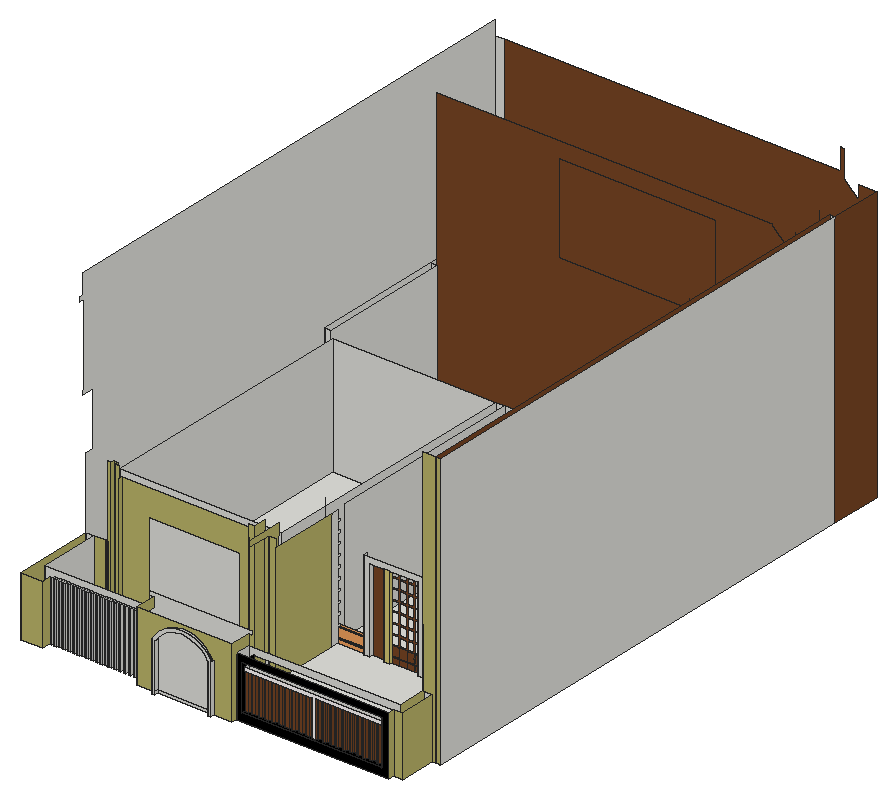
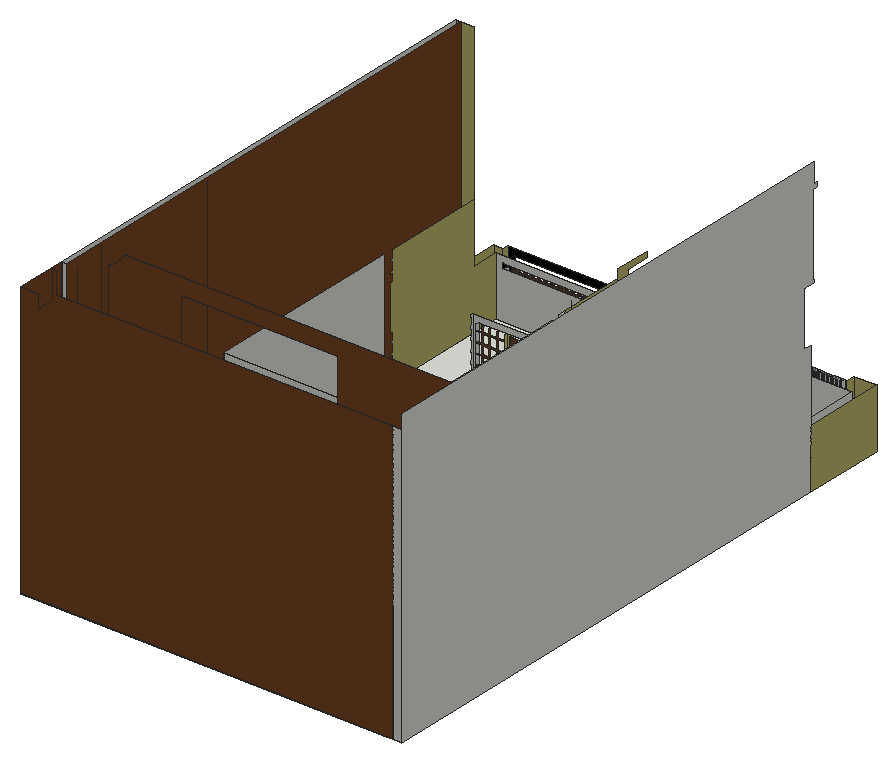
# SketchUp Ruby script. Lengths in inches.
U = 1.inch
M = Sketchup.active_model
def pt(a) = Geom::Point3d.new(a.map { |v| v * U })
def face(e, loops, mat)
  f = e.add_face(loops[0].map { |a| pt(a) })
  loops[1..].each { |l| e.add_face(l.map { |a| pt(a) }).erase! }
  f.material = f.back_material = mat if mat
  f
end
# faces: each face lists its corners as indices into pts; further lists are holes
def faces(e, pts, list, mat = nil) = list.each { |f| face(e, (f[0].is_a?(Array) ? f : [f]).map { |l| l.map { |i| pts[i] } }, mat) }
# xy, xz, yz: faces in a plane at the given z, y or x. An outline is a flat list of corners, or four numbers for a rectangle; further outlines are holes
def ring(l) = l.size == 4 ? [[l[0], l[1]], [l[2], l[1]], [l[2], l[3]], [l[0], l[3]]] : l.each_slice(2).to_a
def flat(e, list, mat, &to3) = list.each { |f| face(e, (f[0].is_a?(Array) ? f : [f]).map { |l| ring(l).map { |u, v| to3.(u, v) } }, mat) }
def xy(e, z, list, mat = nil) = flat(e, list, mat) { |x, y| [x, y, z] }
def xz(e, y, list, mat = nil) = flat(e, list, mat) { |x, z| [x, y, z] }
def yz(e, x, list, mat = nil) = flat(e, list, mat) { |y, z| [x, y, z] }
def lines(e, pts, list) = list.each { |a, b| e.add_line(pt(pts[a]), pt(pts[b])) }
# prism: a flat outline (further loops are holes) pulled along v
def prism(e, loops, v, mat = nil)
  f = face(e, loops, mat); d = Geom::Vector3d.new(v.map { |x| x * U })
  f.pushpull(f.normal.samedirection?(d) ? d.length : -d.length)
end
def box(e, o, s, mat = nil) = prism(e, [[o, [o[0] + s[0], o[1], o[2]], [o[0] + s[0], o[1] + s[1], o[2]], [o[0], o[1] + s[1], o[2]]]], [0, 0, s[2]], mat)
def at(x, y, z, deg = 0) = Geom::Transformation.translation(pt([x, y, z])) * Geom::Transformation.rotation(ORIGIN, Z_AXIS, deg.degrees)
def axes(o, x, y, z) = Geom::Transformation.new([*x, 0, *y, 0, *z, 0, *pt(o).to_a, 1])
def part(name) = M.definitions.add(name)
# library, detail: a bought-in or finely detailed component or shape, given as its bounding box
def library(name, o, s) = part(name).tap { |d| box(d.entities, o, s) }
def detail(e, o, s) = box(e.add_group.entities, o, s)
def put(e, d, t, mat = nil) = e.add_instance(d, t).tap { |i| i.material = mat if mat }
def group(e, t, mat = nil) = e.add_group.tap { |g| g.transformation = t; g.material = mat if mat }.entities
root = M.entities
M.materials.add("[0010_Snow]").color = [255, 250, 250]
M.materials.add("[0037_SandyBrown]").color = [244, 164, 96]
M.materials.add("[0057_DarkKhaki]").color = [189, 183, 107]
M.materials.add("[0131_Silver]").color = [192, 192, 192]
M.materials.add("[0137_Black]").color = [0, 0, 0]
M.materials.add("[Wood Board Cork]").color = [215, 201, 115]
M.materials.add("[Wood Veneer 01]").color = [120, 70, 37]
xy(root,0,[[163.64,1.8125,166.64,1.8125,166.64,4.8125,219.7,4.8125,219.7,1.8125,222.7,1.8125,222.7,4.8125,241.27,4.8125,241.27,25.8125,43.3125,25.8125,43.3125,4.8125,50.69,4.8125,50.69,13.8125,53.49,13.8125,53.49,16.8125,55.32,16.8125,55.32,13.8125,58.12,13.8125,58.12,16.8125,145.98,16.8125,145.98,4.8125,163.64,4.8125],[28.5625,4.8125,28.5625,87.625,36.25,87.625,36.25,25.8125,43.3125,25.8125,43.3125,4.8125],[241.27,10.8125,241.27,25.8125,394.3125,25.8125,394.3125,54.1875,403.3125,54.1875,403.3125,16.8125,394.3125,16.8125,394.3125,10.8125],[59.94,13.8125,62.74,16.8125],[64.57,13.8125,67.37,16.8125],
  [69.19,13.8125,71.99,16.8125],[73.82,13.8125,76.62,16.8125],[78.44,13.8125,81.24,16.8125],[83.07,13.8125,85.87,16.8125],[87.69,13.8125,90.49,16.8125],
  [92.32,13.8125,95.12,16.8125],[96.94,13.8125,99.74,16.8125],[101.57,13.8125,104.37,16.8125],[106.19,13.8125,108.99,16.8125],[110.82,13.8125,113.62,16.8125],
  [115.44,13.8125,118.24,16.8125],[120.07,13.8125,122.87,16.8125],[125.13,13.8125,127.93,16.8125],[130.19,13.8125,132.99,16.8125],[135.25,13.8125,138.06,16.8125],
  [140.32,13.8125,143.12,16.8125],[145.38,13.8125,145.98,16.8125],[36.25,25.8125,43.3125,87.625],[43.3125,25.8125,394.3125,25.8125,394.3125,155.75,314.53,155.75,314.53,154.75,308.53,154.75,308.53,157.75,279.73,157.75,279.73,154.75,274.66,154.75,274.66,157.75,260.53,157.75,260.53,154.75,254.53,154.75,254.53,155.75,227.125,155.75,227.125,77.875,220.06,77.875,220.06,90.625,205.65,90.625,205.65,77.875,199.44,77.875,199.44,90.625,61.7,90.625,61.7,87.625,57.59,87.625,57.59,90.625,53.48,90.625,53.48,87.625,43.3125,87.625],[394.3125,54.1875,395.5625,54.1875,395.5625,376.8125,43.3125,376.8125,43.3125,87.625,47.8125,87.625,47.8125,90.625,50.0625,90.625,50.0625,87.625,53.48,87.625,53.48,90.625,57.59,90.625,57.59,87.625,61.7,87.625,61.7,90.625,199.44,90.625,199.44,77.875,203.15,77.875,203.15,90.625,220.06,90.625,220.06,148.375,225.0625,148.375,225.0625,367.8125,216.0625,367.8125,216.0625,99.625,52.3125,99.625,52.3125,367.8125,394.3125,367.8125],
  [395.5625,54.1875,403.3125,376.8125],[403.3125,54.1875,406.875,376.8125],[406.875,54.1875,410.5,376.8125],[410.5,54.1875,410.5,376.8125,406.875,376.8125,406.875,550.125,410.875,550.125,410.875,54.1875],[410.875,54.1875,411.75,550.125],
  [203.15,77.875,205.65,90.625],[220.06,77.875,225.0625,90.625],[225.0625,77.875,227.125,90.625],[28.5625,87.625,28.5625,601.9375,37.25,601.9375,37.25,376.8125,43.3125,376.8125,43.3125,87.625],[220.06,90.625,225.0625,148.375],
  [225.0625,90.625,227.125,148.375],[52.3125,99.625,216.0625,367.8125],[225.0625,148.375,227.125,157.75],[254.53,154.75,260.53,157.75],[274.66,154.75,279.73,157.75],
  [308.53,154.75,314.53,157.75],[227.125,155.75,254.53,157.75],[314.53,155.75,394.3125,157.75],[225.0625,157.75,394.3125,158.8125],[225.0625,158.8125,394.3125,367.8125],
  [37.25,376.8125,43.3125,510.5],[43.3125,376.8125,395.5625,510.5],[395.5625,376.8125,403.3125,510.5],[403.3125,376.8125,406.875,550.125],[37.25,510.5,43.3125,601.9375],
  [43.3125,510.5,395.5625,550.125],[395.5625,510.5,403.3125,550.125],[43.3125,550.125,403.3125,601.9375],[403.3125,550.125,410.875,601.9375],[410.875,550.125,411.75,601.9375]])
xy(root,3.8125,[[227.125,155.75,254.53,157.75],[314.53,155.75,394.3125,157.75]],"[0037_SandyBrown]")
xy(root,5.97,[[227.125,155.75,254.53,157.75],[314.53,155.75,394.3125,157.75],[227.125,157.75,254.53,157.9375]])
xy(root,7.54,[[246.54,10.8125,387.24,10.8125,387.24,14.8125,385.6,14.8125,385.6,16.8125,381.54,16.8125,381.54,14.8125,378.85,14.8125,378.85,16.8125,374.79,16.8125,374.79,14.8125,372.1,14.8125,372.1,16.8125,368.04,16.8125,368.04,14.8125,365.35,14.8125,365.35,16.8125,361.29,16.8125,361.29,14.8125,358.6,14.8125,358.6,16.8125,354.54,16.8125,354.54,14.8125,351.85,14.8125,351.85,16.8125,347.79,16.8125,347.79,14.8125,345.1,14.8125,345.1,16.8125,341.04,16.8125,341.04,14.8125,338.35,14.8125,338.35,16.8125,334.29,16.8125,334.29,14.8125,331.6,14.8125,331.6,16.8125,327.54,16.8125,327.54,14.8125,324.85,14.8125,324.85,16.8125,320.79,16.8125,320.79,14.8125,318.91,14.8125,318.91,13.8125,314.71,13.8125,314.71,14.8125,314.04,14.8125,314.04,16.8125,311.35,16.8125,311.35,14.8125,307.29,14.8125,307.29,16.8125,304.6,16.8125,304.6,14.8125,300.54,14.8125,300.54,16.8125,297.85,16.8125,297.85,14.8125,293.79,14.8125,293.79,16.8125,291.1,16.8125,291.1,14.8125,287.04,14.8125,287.04,16.8125,284.35,16.8125,284.35,14.8125,280.29,14.8125,280.29,16.8125,277.6,16.8125,277.6,14.8125,273.54,14.8125,273.54,16.8125,270.85,16.8125,270.85,14.8125,266.79,14.8125,266.79,16.8125,264.1,16.8125,264.1,14.8125,260.04,14.8125,260.04,16.8125,257.35,16.8125,257.35,14.8125,253.29,14.8125,253.29,16.8125,250.6,16.8125,250.6,14.8125,246.54,14.8125]],"[0137_Black]")
xy(root,9.66,[[205.65,89.5625,220.06,90.625]])
xy(root,14.375,[[227.125,157.75,254.53,157.9375]])
xy(root,14.375,[[227.125,155.75,254.53,157.75],[314.53,155.75,394.3125,157.75]],"[0037_SandyBrown]")
xz(root,1.8125,[[163.64,0,166.64,0,166.64,48.36,169.3,52.43,173.07,56.4,177.5,59.64,182.43,62.03,187.71,63.5,193.17,63.99,198.63,63.5,203.91,62.03,208.85,59.64,213.27,56.4,217.05,52.43,219.7,48.36,219.7,0,222.7,0,222.7,49.25,219.41,54.29,215.26,58.67,210.4,62.22,204.98,64.85,199.17,66.46,193.17,67,187.17,66.46,181.37,64.85,175.94,62.22,171.08,58.67,166.93,54.29,163.64,49.25]])
xz(root,4.8125,[[166.64,0,219.7,3],[166.64,3,219.7,3,219.7,48.36,217.05,52.43,213.27,56.4,208.85,59.64,203.91,62.03,198.63,63.5,193.17,63.99,187.71,63.5,182.43,62.03,177.5,59.64,173.07,56.4,169.3,52.43,166.64,48.36]])
xz(root,4.8125,[[28.5625,0,50.69,60],[145.98,0,163.64,0,163.64,49.25,166.93,54.29,171.08,58.67,175.94,62.22,181.37,64.85,187.17,66.46,193.17,67,199.17,66.46,204.98,64.85,210.4,62.22,215.26,58.67,219.41,54.29,222.7,49.25,222.7,0,241.27,0,241.27,70.61,145.98,70.61]],"[0057_DarkKhaki]")
xz(root,10.8125,[[[241.27,0,394.3125,60],[246.54,7.54,387.24,53.24]]],"[0137_Black]")
xz(root,13.8125,[[314.71,7.54,318.91,7.54,318.91,44.24,387.24,44.24,387.24,48.11,246.54,48.11,246.54,44.24,314.71,44.24]],"[0010_Snow]")
xz(root,13.8125,[[50.69,0,53.49,60],[55.32,0,58.12,60],[59.94,0,62.74,60],[64.57,0,67.37,60],[69.19,0,71.99,60],
  [73.82,0,76.62,60],[78.44,0,81.24,60],[83.07,0,85.87,60],[87.69,0,90.49,60],[92.32,0,95.12,60],
  [96.94,0,99.74,60],[101.57,0,104.37,60],[106.19,0,108.99,60],[110.82,0,113.62,60],[115.44,0,118.24,60],
  [120.07,0,122.87,60],[125.13,0,127.93,60],[130.19,0,132.99,60],[135.25,0,138.06,60],[140.32,0,143.12,60],
  [145.38,0,145.98,60]],"[0131_Silver]")
xz(root,14.8125,[[246.54,7.54,250.6,44.24],[253.29,7.54,257.35,44.24],[260.04,7.54,264.1,44.24],[266.79,7.54,270.85,44.24],[273.54,7.54,277.6,44.24],
  [280.29,7.54,284.35,44.24],[287.04,7.54,291.1,44.24],[293.79,7.54,297.85,44.24],[300.54,7.54,304.6,44.24],[307.29,7.54,311.35,44.24],
  [314.04,7.54,314.71,44.24],[318.91,7.54,320.79,44.24],[324.85,7.54,327.54,44.24],[331.6,7.54,334.29,44.24],[338.35,7.54,341.04,44.24],
  [345.1,7.54,347.79,44.24],[351.85,7.54,354.54,44.24],[358.6,7.54,361.29,44.24],[365.35,7.54,368.04,44.24],[372.1,7.54,374.79,44.24],
  [378.85,7.54,381.54,44.24],[385.6,7.54,387.24,44.24]],"[Wood Veneer 01]")
xz(root,16.8125,[[59.94,0,62.74,60],[64.57,0,67.37,60],[69.19,0,71.99,60],[73.82,0,76.62,60],[78.44,0,81.24,60],
  [83.07,0,85.87,60],[87.69,0,90.49,60],[92.32,0,95.12,60],[96.94,0,99.74,60],[101.57,0,104.37,60],
  [106.19,0,108.99,60],[110.82,0,113.62,60],[115.44,0,118.24,60],[120.07,0,122.87,60],[125.13,0,127.93,60],
  [130.19,0,132.99,60],[135.25,0,138.06,60],[140.32,0,143.12,60],[145.38,0,145.98,60],[145.98,0,148.18,60],
  [314.71,7.54,318.1,44.24],[388.29,7.54,392.35,44.24]])
xz(root,16.8125,[[394.3125,0,403.3125,60]],"[0057_DarkKhaki]")
xz(root,16.8125,[[53.49,0,55.32,60],[58.12,0,59.94,60],[62.74,0,64.57,60],[67.37,0,69.19,60],[71.99,0,73.82,60],
  [76.62,0,78.44,60],[81.24,0,83.07,60],[85.87,0,87.69,60],[90.49,0,92.32,60],[95.12,0,96.94,60],
  [99.74,0,101.57,60],[104.37,0,106.19,60],[108.99,0,110.82,60],[113.62,0,115.44,60],[118.24,0,120.07,60],
  [122.87,0,125.13,60],[127.93,0,130.19,60],[132.99,0,135.25,60],[138.06,0,140.32,60],[143.12,0,145.38,60]],"[0131_Silver]")
xz(root,16.8125,[[250.6,7.54,253.29,44.24],[257.35,7.54,260.04,44.24],[264.1,7.54,266.79,44.24],[270.85,7.54,273.54,44.24],[277.6,7.54,280.29,44.24],
  [284.35,7.54,287.04,44.24],[291.1,7.54,293.79,44.24],[297.85,7.54,300.54,44.24],[304.6,7.54,307.29,44.24],[311.35,7.54,314.04,44.24],
  [320.79,7.54,324.85,44.24],[327.54,7.54,331.6,44.24],[334.29,7.54,338.35,44.24],[341.04,7.54,345.1,44.24],[347.79,7.54,351.85,44.24],
  [354.54,7.54,358.6,44.24],[361.29,7.54,365.35,44.24],[368.04,7.54,372.1,44.24],[374.79,7.54,378.85,44.24],[381.54,7.54,385.6,44.24]],"[Wood Veneer 01]")
xz(root,25.8125,[[36.25,0,36.25,60,145.98,60,145.98,70.61,142.42,70.61,142.42,74.1875,244.96,74.1875,244.96,70.75,241.27,70.75,241.27,0],[[241.27,0,394.3125,60],[246.54,48.11,387.24,53.24]]])
xz(root,54.1875,[[395.5625,0,403.3125,60]])
xz(root,54.1875,[[403.3125,0,406.875,0,406.875,276,394.3125,276,394.3125,60,403.3125,60],[406.875,0,411.75,276]],"[0057_DarkKhaki]")
xz(root,77.875,[[199.44,0,205.65,132],[220.06,0,227.125,128.6875]],"[0057_DarkKhaki]")
xz(root,87.625,[[28.5625,0,36.25,60]])
xz(root,87.625,[[36.25,0,47.8125,60],[47.8125,0,50.0625,60],[50.0625,0,53.48,132],[57.59,0,61.7,132]],"[0057_DarkKhaki]")
xz(root,89.5625,[[205.65,9.66,220.06,123.17]],"[0057_DarkKhaki]")
xz(root,90.625,[[47.8125,0,50.0625,60],[205.65,0,220.06,9.66]])
xz(root,90.625,[[53.48,0,57.59,132],[[61.7,0,199.44,120],[88.6875,15.35,180.5,93.6]]],"[0057_DarkKhaki]")
xz(root,99.625,[[52.3125,0,216.0625,120]])
xz(root,154.75,[[254.53,0,260.53,0,260.53,84,308.53,84,308.53,0,314.53,0,314.53,90,254.53,90]])
xz(root,154.75,[[274.66,0,279.73,84]],"[Wood Board Cork]")
xz(root,155.75,[[227.125,0,254.53,3.8125],[314.53,0,394.3125,3.8125],[227.125,5.97,254.53,14.375],[314.53,5.97,394.3125,14.375]],"[0037_SandyBrown]")
xz(root,157.75,[[225.0625,0,227.125,3.8125],[227.125,0,254.53,3.8125],[254.53,0,260.53,3.8125],[274.66,0,279.73,3.8125],[308.53,0,314.53,3.8125],
  [314.53,0,394.3125,3.8125],[225.0625,3.8125,227.125,5.97],[254.53,3.8125,260.53,5.97],[308.53,3.8125,314.53,5.97],[225.0625,5.97,227.125,14.375],
  [254.53,5.97,260.53,14.375],[274.66,5.97,279.73,14.375],[308.53,5.97,314.53,14.375],[314.53,5.97,394.3125,14.375],[225.0625,14.375,227.125,16.53],
  [254.53,14.375,260.53,16.53],[308.53,14.375,314.53,16.53]])
xz(root,157.75,[[227.125,3.8125,254.53,5.97],[314.53,3.8125,394.3125,5.97],[227.125,14.375,254.53,16.53],[314.53,14.375,394.3125,16.53]],"[0037_SandyBrown]")
xz(root,157.75,[[260.53,0,274.66,84],[279.73,0,286.72,5.28],[[286.72,0,287.41,0,287.41,5.28,295.09,5.28,295.09,0,295.95,0,295.95,5.28,302.05,5.28,302.05,0,302.96,0,302.96,5.28,308.53,5.28,308.53,6.47,302.96,6.47,302.96,15.84,308.53,15.84,308.53,17.03,302.96,17.03,302.96,25.59,308.53,25.59,308.53,26.78,302.96,26.78,302.96,35.97,308.53,35.97,308.53,37.15,302.96,37.15,302.96,46.34,308.53,46.34,308.53,47.53,302.96,47.53,302.96,56.72,308.53,56.72,308.53,57.9,302.96,57.9,302.96,67.09,308.53,67.09,308.53,68.28,302.96,68.28,302.96,77.47,308.53,77.47,308.53,78.65,302.96,78.65,302.96,84,302.05,84,302.05,78.65,295.95,78.65,295.95,84,295.09,84,295.09,78.65,287.41,78.65,287.41,84,286.72,84,286.72,78.65,279.73,78.65,279.73,77.47,286.72,77.47,286.72,68.28,279.73,68.28,279.73,67.09,286.72,67.09,286.72,57.9,279.73,57.9,279.73,56.72,286.72,56.72,286.72,47.53,279.73,47.53,279.73,46.34,286.72,46.34,286.72,37.15,279.73,37.15,279.73,35.97,286.72,35.97,286.72,26.78,279.73,26.78,279.73,25.59,286.72,25.59,286.72,17.03,279.73,17.03,279.73,15.84,286.72,15.84,286.72,6.47,279.73,6.47,279.73,5.28,286.72,5.28],[287.41,6.47,295.09,15.84],[287.41,68.28,295.09,77.47],[287.41,26.78,295.09,35.97],[287.41,47.53,295.09,56.72],[287.41,57.9,295.09,67.09],[287.41,37.15,295.09,46.34],[287.41,17.03,295.09,25.59],[295.95,6.47,302.05,15.84],[295.95,68.28,302.05,77.47],[295.95,26.78,302.05,35.97],[295.95,47.53,302.05,56.72],[295.95,57.9,302.05,67.09],[295.95,37.15,302.05,46.34],[295.95,17.03,302.05,25.59]],[287.41,0,295.09,5.28],[295.95,0,302.05,5.28],
  [302.96,0,308.53,5.28],[279.73,6.47,286.72,15.84],[287.41,6.47,295.09,15.84],[295.95,6.47,302.05,15.84],[302.96,6.47,308.53,15.84]],"[Wood Veneer 01]")
xz(root,157.9375,[[227.125,5.97,254.53,14.375]])
xz(root,367.8125,[[52.3125,0,216.0625,120],[216.0625,0,225.0625,120],[225.0625,0,394.3125,120]])
xz(root,376.8125,[[37.25,0,43.3125,120]])
xz(root,510.5,[[37.25,0,43.3125,120]])
xz(root,510.5,[[[43.3125,0,395.5625,0,395.5625,262.35,394.3125,261.1,393.87,260.66,378.97,275.56,379.41,276,43.3125,276],[165.9,169.8,323.53,259.87]]],"[Wood Veneer 01]")
xz(root,550.125,[[406.875,0,411.75,276]])
xz(root,601.9375,[[28.5625,0,37.25,281.9375]])
xz(root,601.9375,[[37.25,0,37.25,281.9375,375.74,281.9375,375.74,303.3125,379.41,303.3125,379.41,297.01,378.88,297.01,379.41,296.54,379.41,276,394.3125,261.1,394.3125,276,411.75,276,411.75,0]],"[Wood Veneer 01]")
yz(root,28.5625,[[87.625,0,87.625,132,95.4375,132,95.4375,186.28,82.875,186.28,82.875,189.28,85.1875,189.28,85.1875,271.48,79.4375,271.48,79.4375,276,83.625,276,83.625,295.8125,601.9375,295.8125,601.9375,0]])
yz(root,28.5625,[[4.8125,0,87.625,60]],"[0057_DarkKhaki]")
yz(root,36.25,[[25.8125,0,87.625,60]])
yz(root,37.25,[[376.8125,0,510.5,120],[510.5,0,601.9375,120]])
yz(root,43.3125,[[376.8125,0,510.5,120]])
yz(root,47.8125,[[87.625,0,90.625,60]])
yz(root,50.0625,[[87.625,0,90.625,60]])
yz(root,50.69,[[4.8125,0,13.8125,60]],"[0057_DarkKhaki]")
yz(root,52.3125,[[99.625,0,367.8125,120]])
yz(root,53.48,[[87.625,0,90.625,132]],"[0057_DarkKhaki]")
yz(root,53.49,[[13.8125,0,16.8125,60]])
yz(root,55.32,[[13.8125,0,16.8125,60]])
yz(root,57.59,[[87.625,0,90.625,132]],"[0057_DarkKhaki]")
yz(root,58.12,[[13.8125,0,16.8125,60]])
yz(root,59.94,[[13.8125,0,16.8125,60]])
yz(root,61.7,[[87.625,0,90.625,120]],"[0057_DarkKhaki]")
yz(root,62.74,[[13.8125,0,16.8125,60]])
yz(root,64.57,[[13.8125,0,16.8125,60]])
yz(root,67.37,[[13.8125,0,16.8125,60]])
yz(root,69.19,[[13.8125,0,16.8125,60]])
yz(root,71.99,[[13.8125,0,16.8125,60]])
yz(root,73.82,[[13.8125,0,16.8125,60]])
yz(root,76.62,[[13.8125,0,16.8125,60]])
yz(root,78.44,[[13.8125,0,16.8125,60]])
yz(root,81.24,[[13.8125,0,16.8125,60]])
yz(root,83.07,[[13.8125,0,16.8125,60]],"[0131_Silver]")
yz(root,85.87,[[13.8125,0,16.8125,60]])
yz(root,87.69,[[13.8125,0,16.8125,60]],"[0131_Silver]")
yz(root,90.49,[[13.8125,0,16.8125,60]])
yz(root,92.32,[[13.8125,0,16.8125,60]])
yz(root,95.12,[[13.8125,0,16.8125,60]])
yz(root,96.94,[[13.8125,0,16.8125,60]])
yz(root,99.74,[[13.8125,0,16.8125,60]])
yz(root,101.57,[[13.8125,0,16.8125,60]])
yz(root,104.37,[[13.8125,0,16.8125,60]])
yz(root,106.19,[[13.8125,0,16.8125,60]],"[0131_Silver]")
yz(root,108.99,[[13.8125,0,16.8125,60]])
yz(root,110.82,[[13.8125,0,16.8125,60]])
yz(root,113.62,[[13.8125,0,16.8125,60]])
yz(root,115.44,[[13.8125,0,16.8125,60]])
yz(root,118.24,[[13.8125,0,16.8125,60]])
yz(root,120.07,[[13.8125,0,16.8125,60]])
yz(root,122.87,[[13.8125,0,16.8125,60]])
yz(root,125.13,[[13.8125,0,16.8125,60]])
yz(root,127.93,[[13.8125,0,16.8125,60]])
yz(root,130.19,[[13.8125,0,16.8125,60]])
yz(root,132.99,[[13.8125,0,16.8125,60]])
yz(root,135.25,[[13.8125,0,16.8125,60]])
yz(root,138.06,[[13.8125,0,16.8125,60]])
yz(root,140.32,[[13.8125,0,16.8125,60]])
yz(root,143.12,[[13.8125,0,16.8125,60]])
yz(root,145.38,[[13.8125,0,16.8125,60]])
yz(root,145.98,[[13.8125,0,16.8125,60]])
yz(root,145.98,[[4.8125,0,4.8125,70.61,25.8125,70.61,25.8125,60,13.8125,60,13.8125,0]],"[0057_DarkKhaki]")
yz(root,163.64,[[1.8125,0,4.8125,49.25]])
yz(root,166.64,[[1.8125,0,4.8125,3],[1.8125,3,4.8125,48.36]])
yz(root,199.44,[[77.875,0,90.625,120]],"[0057_DarkKhaki]")
yz(root,205.65,[[77.875,0,90.625,0,90.625,9.66,89.5625,9.66,89.5625,123.17,90.625,123.17,90.625,132,77.875,132]],"[0057_DarkKhaki]")
yz(root,216.0625,[[99.625,0,367.8125,120]])
yz(root,219.7,[[1.8125,0,4.8125,3],[1.8125,3,4.8125,48.36]])
yz(root,220.06,[[77.875,0,77.875,128.6875,54.1875,128.6875,54.1875,134.75,90.625,134.75,90.625,123.17,89.5625,123.17,89.5625,9.66,90.625,9.66,90.625,0]],"[0057_DarkKhaki]")
yz(root,222.7,[[1.8125,0,4.8125,49.25]])
yz(root,225.0625,[[166.75,0,367.8125,120]])
yz(root,227.125,[[148.375,0,155.75,0,155.75,3.8125,157.75,3.8125,157.75,5.97,155.75,5.97,155.75,14.375,157.75,14.375,157.75,16.53,155.75,16.53,155.75,24.9375,157.75,24.9375,157.75,27.1,155.75,27.1,155.75,35.5,157.75,35.5,157.75,37.66,155.75,37.66,155.75,46.0625,157.75,46.0625,157.75,48.22,155.75,48.22,155.75,56.625,157.75,56.625,157.75,58.78,155.75,58.78,155.75,67.1875,157.75,67.1875,157.75,69.35,155.75,69.35,155.75,77.75,157.75,77.75,157.75,79.91,155.75,79.91,155.75,88.3125,157.75,88.3125,157.75,90.47,155.75,90.47,155.75,98.875,157.75,98.875,157.75,101.03,155.75,101.03,155.75,109.4375,157.75,109.4375,157.75,111.6,155.75,111.6,155.75,120,148.375,120],[155.75,0,157.75,3.8125],[155.75,5.97,157.75,14.375],[157.75,5.97,157.9375,14.375]])
yz(root,227.125,[[77.875,0,148.375,120]],"[0057_DarkKhaki]")
yz(root,241.27,[[10.8125,0,25.8125,60]])
yz(root,241.27,[[4.8125,0,10.8125,0,10.8125,60,25.8125,60,25.8125,70.61,4.8125,70.61]],"[0057_DarkKhaki]")
yz(root,246.54,[[10.8125,7.54,14.8125,7.54,14.8125,44.24,13.8125,44.24,13.8125,48.11,25.8125,48.11,25.8125,53.24,10.8125,53.24]],"[0137_Black]")
yz(root,250.6,[[14.8125,7.54,16.8125,44.24]],"[Wood Veneer 01]")
yz(root,253.29,[[14.8125,7.54,16.8125,44.24]],"[Wood Veneer 01]")
yz(root,254.53,[[154.75,0,154.75,90,157.75,90,157.75,88.3125,155.75,88.3125,155.75,79.91,157.75,79.91,157.75,77.75,155.75,77.75,155.75,69.35,157.75,69.35,157.75,67.1875,155.75,67.1875,155.75,58.78,157.75,58.78,157.75,56.625,155.75,56.625,155.75,48.22,157.75,48.22,157.75,46.0625,155.75,46.0625,155.75,37.66,157.75,37.66,157.75,35.5,155.75,35.5,155.75,27.1,157.75,27.1,157.75,24.9375,155.75,24.9375,155.75,16.53,157.75,16.53,157.75,14.375,155.75,14.375,155.75,5.97,157.75,5.97,157.75,3.8125,155.75,3.8125,155.75,0],[155.75,0,157.75,3.8125],[155.75,5.97,157.75,14.375],[157.75,5.97,157.9375,14.375]])
yz(root,257.35,[[14.8125,7.54,16.8125,44.24]],"[Wood Veneer 01]")
yz(root,260.04,[[14.8125,7.54,16.8125,44.24]],"[Wood Veneer 01]")
yz(root,260.53,[[154.75,0,157.75,84]])
yz(root,264.1,[[14.8125,7.54,16.8125,44.24]],"[Wood Veneer 01]")
yz(root,266.79,[[14.8125,7.54,16.8125,44.24]],"[Wood Veneer 01]")
yz(root,270.85,[[14.8125,7.54,16.8125,44.24]],"[Wood Veneer 01]")
yz(root,273.54,[[14.8125,7.54,16.8125,44.24]],"[Wood Veneer 01]")
yz(root,274.66,[[154.75,0,157.75,84]],"[Wood Board Cork]")
yz(root,277.6,[[14.8125,7.54,16.8125,44.24]],"[Wood Veneer 01]")
yz(root,279.73,[[154.75,0,157.75,84]],"[Wood Board Cork]")
yz(root,280.29,[[14.8125,7.54,16.8125,44.24]],"[Wood Veneer 01]")
yz(root,284.35,[[14.8125,7.54,16.8125,44.24]],"[Wood Veneer 01]")
yz(root,287.04,[[14.8125,7.54,16.8125,44.24]],"[Wood Veneer 01]")
yz(root,291.1,[[14.8125,7.54,16.8125,44.24]],"[Wood Veneer 01]")
yz(root,293.79,[[14.8125,7.54,16.8125,44.24]],"[Wood Veneer 01]")
yz(root,297.85,[[14.8125,7.54,16.8125,44.24]],"[Wood Veneer 01]")
yz(root,300.54,[[14.8125,7.54,16.8125,44.24]],"[Wood Veneer 01]")
yz(root,304.6,[[14.8125,7.54,16.8125,44.24]],"[Wood Veneer 01]")
yz(root,307.29,[[14.8125,7.54,16.8125,44.24]],"[Wood Veneer 01]")
yz(root,308.53,[[154.75,0,157.75,84]])
yz(root,311.35,[[14.8125,7.54,16.8125,44.24]],"[Wood Veneer 01]")
yz(root,314.04,[[14.8125,7.54,16.8125,44.24]],"[Wood Veneer 01]")
yz(root,314.53,[[154.75,0,155.75,0,155.75,3.8125,157.75,3.8125,157.75,5.97,155.75,5.97,155.75,14.375,157.75,14.375,157.75,16.53,155.75,16.53,155.75,24.9375,157.75,24.9375,157.75,27.1,155.75,27.1,155.75,35.5,157.75,35.5,157.75,37.66,155.75,37.66,155.75,46.0625,157.75,46.0625,157.75,48.22,155.75,48.22,155.75,56.625,157.75,56.625,157.75,58.78,155.75,58.78,155.75,67.1875,157.75,67.1875,157.75,69.35,155.75,69.35,155.75,77.75,157.75,77.75,157.75,79.91,155.75,79.91,155.75,88.3125,157.75,88.3125,157.75,90,154.75,90],[155.75,0,157.75,3.8125],[155.75,5.97,157.75,14.375]])
yz(root,314.71,[[14.8125,7.54,16.8125,44.24]])
yz(root,314.71,[[13.8125,7.54,14.8125,44.24]],"[Wood Veneer 01]")
yz(root,318.91,[[13.8125,7.54,14.8125,44.24]],"[Wood Veneer 01]")
yz(root,320.79,[[14.8125,7.54,16.8125,44.24]],"[Wood Veneer 01]")
yz(root,324.85,[[14.8125,7.54,16.8125,44.24]],"[Wood Veneer 01]")
yz(root,327.54,[[14.8125,7.54,16.8125,44.24]],"[Wood Veneer 01]")
yz(root,331.6,[[14.8125,7.54,16.8125,44.24]],"[Wood Veneer 01]")
yz(root,334.29,[[14.8125,7.54,16.8125,44.24]],"[Wood Veneer 01]")
yz(root,338.35,[[14.8125,7.54,16.8125,44.24]],"[Wood Veneer 01]")
yz(root,341.04,[[14.8125,7.54,16.8125,44.24]],"[Wood Veneer 01]")
yz(root,345.1,[[14.8125,7.54,16.8125,44.24]],"[Wood Veneer 01]")
yz(root,347.79,[[14.8125,7.54,16.8125,44.24]],"[Wood Veneer 01]")
yz(root,351.85,[[14.8125,7.54,16.8125,44.24]],"[Wood Veneer 01]")
yz(root,354.54,[[14.8125,7.54,16.8125,44.24]],"[Wood Veneer 01]")
yz(root,358.6,[[14.8125,7.54,16.8125,44.24]],"[Wood Veneer 01]")
yz(root,361.29,[[14.8125,7.54,16.8125,44.24]],"[Wood Veneer 01]")
yz(root,365.35,[[14.8125,7.54,16.8125,44.24]],"[Wood Veneer 01]")
yz(root,368.04,[[14.8125,7.54,16.8125,44.24]],"[Wood Veneer 01]")
yz(root,372.1,[[14.8125,7.54,16.8125,44.24]],"[Wood Veneer 01]")
yz(root,374.79,[[14.8125,7.54,16.8125,44.24]],"[Wood Veneer 01]")
yz(root,378.85,[[14.8125,7.54,16.8125,44.24]],"[Wood Veneer 01]")
yz(root,381.54,[[14.8125,7.54,16.8125,44.24]],"[Wood Veneer 01]")
yz(root,385.6,[[14.8125,7.54,16.8125,44.24]],"[Wood Veneer 01]")
yz(root,387.24,[[10.8125,7.54,10.8125,53.24,25.8125,53.24,25.8125,48.11,13.8125,48.11,13.8125,44.24,14.8125,44.24,14.8125,7.54]],"[0137_Black]")
yz(root,394.3125,[[155.75,0,157.75,3.8125],[166.75,0,367.8125,120],[155.75,5.97,157.75,14.375]])
yz(root,394.3125,[[10.8125,0,16.8125,60],[25.8125,0,25.8125,60,54.1875,60,54.1875,120,155.75,120,155.75,111.6,157.75,111.6,157.75,109.4375,155.75,109.4375,155.75,101.03,157.75,101.03,157.75,98.875,155.75,98.875,155.75,90.47,157.75,90.47,157.75,46.0625,155.75,46.0625,155.75,37.66,157.75,37.66,157.75,35.5,155.75,35.5,155.75,27.1,157.75,27.1,157.75,24.9375,155.75,24.9375,155.75,16.53,157.75,16.53,157.75,14.375,155.75,14.375,155.75,5.97,157.75,5.97,157.75,3.8125,155.75,3.8125,155.75,0]],"[0057_DarkKhaki]")
yz(root,403.3125,[[16.8125,0,54.1875,60]],"[0057_DarkKhaki]")
yz(root,406.875,[[54.1875,0,550.125,276]],"[Wood Veneer 01]")
yz(root,411.75,[[54.1875,0,550.125,276]])
yz(root,411.75,[[550.125,0,601.9375,276]],"[Wood Veneer 01]")
p = [[403.3125,376.8125,0],[403.3125,376.8125,276],[225.0625,158.8125,0],[224.5625,158.8125,0],[220.06,148.375,0],[220.06,148.375,132],
  [403.3125,510.5,0],[403.3125,510.5,276],[395.5625,550.125,0],[395.5625,550.125,276]]
lines(root,p,[[0,1],[2,3],[4,5],[6,7],[8,9]])
